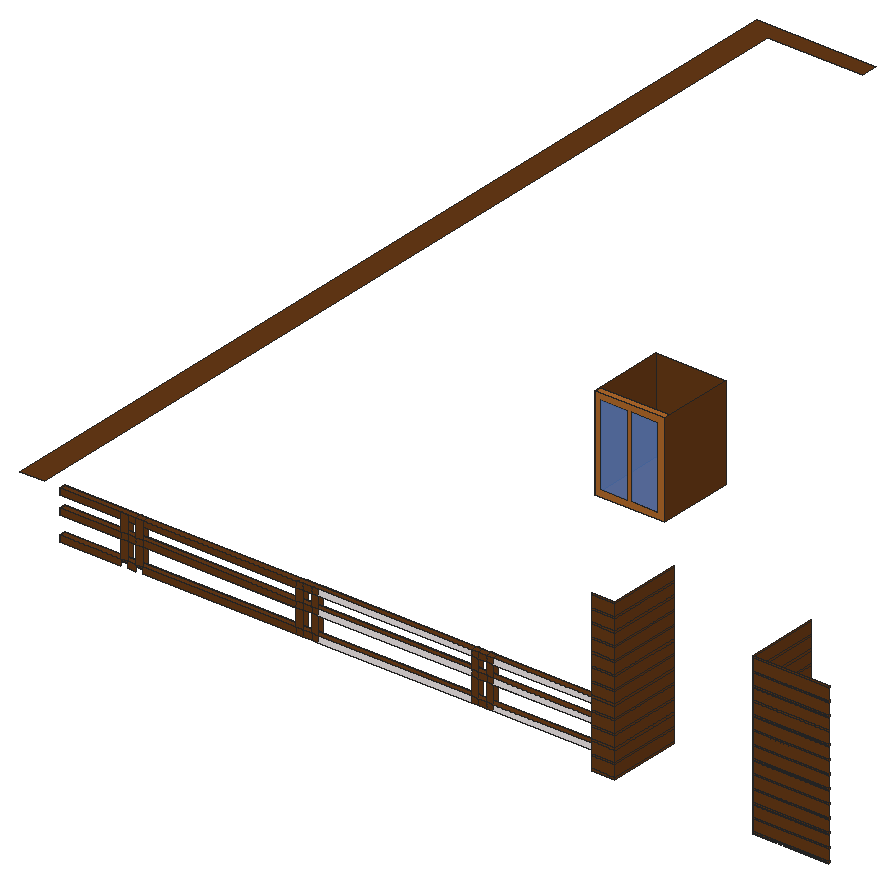
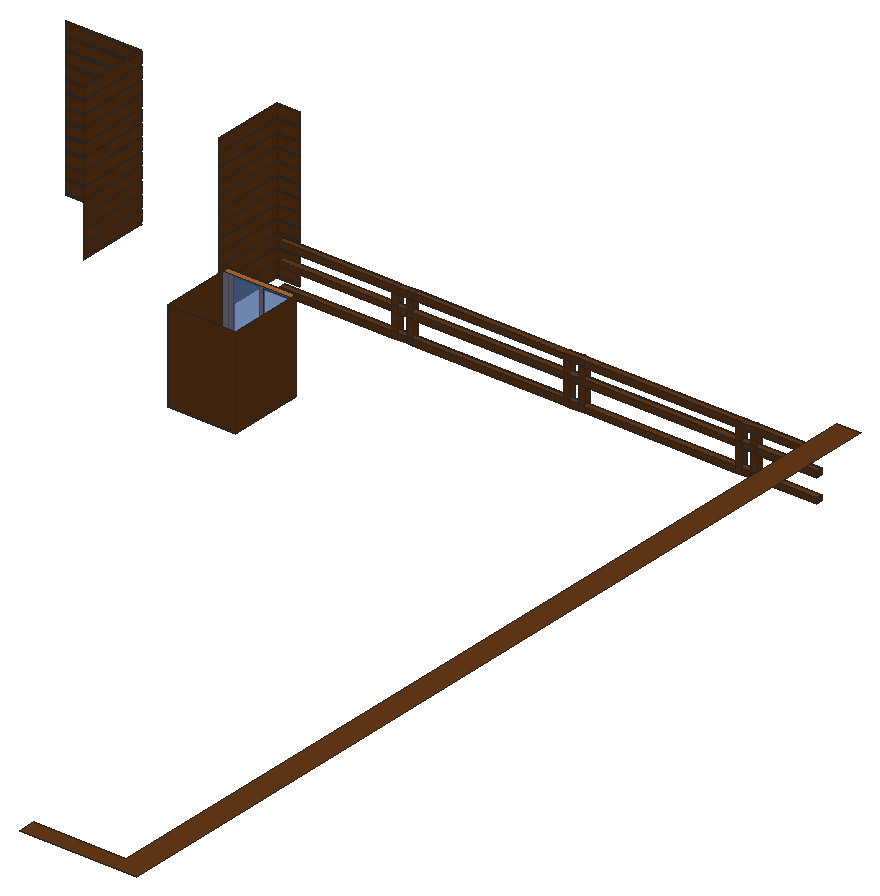
# SketchUp Ruby script. Lengths in inches.
U = 1.inch
M = Sketchup.active_model
def pt(a) = Geom::Point3d.new(a.map { |v| v * U })
def face(e, loops, mat)
  f = e.add_face(loops[0].map { |a| pt(a) })
  loops[1..].each { |l| e.add_face(l.map { |a| pt(a) }).erase! }
  f.material = f.back_material = mat if mat
  f
end
# faces: each face lists its corners as indices into pts; further lists are holes
def faces(e, pts, list, mat = nil) = list.each { |f| face(e, (f[0].is_a?(Array) ? f : [f]).map { |l| l.map { |i| pts[i] } }, mat) }
# xy, xz, yz: faces in a plane at the given z, y or x. An outline is a flat list of corners, or four numbers for a rectangle; further outlines are holes
def ring(l) = l.size == 4 ? [[l[0], l[1]], [l[2], l[1]], [l[2], l[3]], [l[0], l[3]]] : l.each_slice(2).to_a
def flat(e, list, mat, &to3) = list.each { |f| face(e, (f[0].is_a?(Array) ? f : [f]).map { |l| ring(l).map { |u, v| to3.(u, v) } }, mat) }
def xy(e, z, list, mat = nil) = flat(e, list, mat) { |x, y| [x, y, z] }
def xz(e, y, list, mat = nil) = flat(e, list, mat) { |x, z| [x, y, z] }
def yz(e, x, list, mat = nil) = flat(e, list, mat) { |y, z| [x, y, z] }
def lines(e, pts, list) = list.each { |a, b| e.add_line(pt(pts[a]), pt(pts[b])) }
# prism: a flat outline (further loops are holes) pulled along v
def prism(e, loops, v, mat = nil)
  f = face(e, loops, mat); d = Geom::Vector3d.new(v.map { |x| x * U })
  f.pushpull(f.normal.samedirection?(d) ? d.length : -d.length)
end
def box(e, o, s, mat = nil) = prism(e, [[o, [o[0] + s[0], o[1], o[2]], [o[0] + s[0], o[1] + s[1], o[2]], [o[0], o[1] + s[1], o[2]]]], [0, 0, s[2]], mat)
def at(x, y, z, deg = 0) = Geom::Transformation.translation(pt([x, y, z])) * Geom::Transformation.rotation(ORIGIN, Z_AXIS, deg.degrees)
def axes(o, x, y, z) = Geom::Transformation.new([*x, 0, *y, 0, *z, 0, *pt(o).to_a, 1])
def part(name) = M.definitions.add(name)
# library, detail: a bought-in or finely detailed component or shape, given as its bounding box
def library(name, o, s) = part(name).tap { |d| box(d.entities, o, s) }
def detail(e, o, s) = box(e.add_group.entities, o, s)
def put(e, d, t, mat = nil) = e.add_instance(d, t).tap { |i| i.material = mat if mat }
def group(e, t, mat = nil) = e.add_group.tap { |g| g.transformation = t; g.material = mat if mat }.entities
root = M.entities
M.materials.add("Generic").color = [102, 57, 22]
M.materials.add("Generic\#3").color = [243, 235, 235]
M.materials.add("[Translucent Glass Blue]1").color = [100, 149, 237]
M.materials["[Translucent Glass Blue]1"].alpha = 0.5
M.materials.add("[Wood Bamboo]").color = [177, 105, 43]
c1 = part("Group\#5")
xy(c1.entities,0,[[0,0,33.5625,3]],"[Wood Bamboo]")
xy(c1.entities,44.875,[[0,0,33.5625,3]],"[Wood Bamboo]")
xz(c1.entities,0,[[3.04,3.04,15.78,41.84],[17.78,3.04,30.53,41.84]],"[Translucent Glass Blue]1")
xz(c1.entities,0,[[[0,0,33.5625,44.875],[3.04,3.04,15.78,41.84],[17.78,3.04,30.53,41.84]]],"[Wood Bamboo]")
xz(c1.entities,3,[[0,0,33.5625,44.875]],"[Translucent Glass Blue]1")
yz(c1.entities,0,[[0,0,3,44.875]],"[Wood Bamboo]")
yz(c1.entities,33.5625,[[0,0,3,44.875]],"[Wood Bamboo]")
xy(root,296,[[366.12,54.375,377.375,54.68],[377.375,54.375,403,54.68]],"Generic")
xy(root,297,[[366.12,54.375,377.375,54.68],[377.375,54.375,403,54.68]],"Generic")
xy(root,302.3125,[[366.12,54.375,377.375,54.68],[377.375,54.375,403,54.68]],"Generic")
xy(root,303.3125,[[366.12,54.375,377.375,54.68],[377.375,54.375,403,54.68]],"Generic")
xy(root,308.625,[[366.12,54.375,377.375,54.68],[377.375,54.375,403,54.68]],"Generic")
xy(root,309.625,[[366.12,54.375,377.375,54.68],[377.375,54.375,403,54.68]],"Generic")
xy(root,314.9375,[[366.12,54.375,377.375,54.68],[377.375,54.375,403,54.68]],"Generic")
xy(root,315.9375,[[366.12,54.375,377.375,54.68],[377.375,54.375,403,54.68]],"Generic")
xy(root,321.25,[[366.12,54.375,377.375,54.68],[377.375,54.375,403,54.68]],"Generic")
xy(root,321.29,[[54.37,63.57,57.43,66.56],[138.81,63.57,141.87,66.56],[146.12,63.57,149.18,66.56]],"Generic")
xy(root,321.32,[[61.68,63.57,64.75,66.56],[223.25,63.57,226.31,66.56],[230.56,63.57,233.62,66.56]],"Generic")
xy(root,322.25,[[366.12,54.375,377.375,54.68],[377.375,54.375,403,54.68]],"Generic")
xy(root,327.5625,[[366.12,54.375,377.375,54.68],[377.375,54.375,403,54.68]],"Generic")
xy(root,328.375,[[13.1875,54.375,25.02,54.375,25.02,490.0625,70.5625,490.0625,70.5625,498.375,13.1875,498.375]],"Generic")
xy(root,328.5625,[[366.12,54.375,377.375,54.68],[377.375,54.375,403,54.68]],"Generic")
xy(root,331.3125,[[196.46,171.5,230.03,208.375]],"Generic")
xy(root,333.875,[[366.12,54.375,377.375,54.68],[377.375,54.375,403,54.68]],"Generic")
xy(root,334.875,[[366.12,54.375,377.375,54.68],[377.375,54.375,403,54.68]],"Generic")
xy(root,340.1875,[[366.12,54.375,377.375,54.68],[377.375,54.375,403,54.68]],"Generic")
xy(root,341.1875,[[366.12,54.375,377.375,54.68],[377.375,54.375,403,54.68]],"Generic")
xy(root,346.5,[[366.12,54.375,377.375,54.68],[377.375,54.375,403,54.68]],"Generic")
xy(root,347.5,[[366.12,54.375,377.375,54.68],[377.375,54.375,403,54.68]],"Generic")
xy(root,359.125,[[366.12,54.375,377.375,54.68],[377.375,54.375,403,54.68]],"Generic")
xy(root,360.125,[[366.12,54.375,377.375,54.68],[377.375,54.375,403,54.68]],"Generic")
xy(root,365.4375,[[366.12,54.375,377.375,54.68],[377.375,54.375,403,54.68]],"Generic")
xy(root,366.4375,[[366.12,54.375,377.375,54.68],[377.375,54.375,403,54.68]],"Generic")
xy(root,371.75,[[366.12,54.375,377.375,54.68],[377.375,54.375,403,54.68]],"Generic")
xz(root,54.375,[[288.56,296,299.81,297],[288.56,297,299.81,302.3125],[366.12,297,403,302.3125],[288.56,302.3125,299.81,303.3125],[288.56,303.3125,299.81,308.625],
  [366.12,303.3125,403,308.625],[288.56,308.625,299.81,309.625],[288.56,309.625,299.81,314.9375],[366.12,309.625,403,314.9375],[288.56,314.9375,299.81,315.9375],
  [288.56,315.9375,299.81,321.25],[366.12,315.9375,403,321.25],[288.56,321.25,299.81,322.25],[288.56,322.25,299.81,327.5625],[366.12,322.25,403,327.5625],
  [288.56,327.5625,299.81,328.5625],[288.56,328.5625,299.81,333.875],[366.12,328.5625,403,333.875],[288.56,333.875,299.81,334.875],[288.56,334.875,299.81,340.1875],
  [366.12,334.875,403,340.1875],[288.56,340.1875,299.81,341.1875],[288.56,341.1875,299.81,346.5],[366.12,341.1875,403,346.5],[288.56,346.5,299.81,347.5],
  [288.56,347.5,299.81,352.8125],[366.12,347.5,403,352.8125],[288.56,352.8125,299.81,353.8125],[366.12,352.8125,403,353.8125],[288.56,353.8125,299.81,359.125],
  [366.12,353.8125,403,359.125],[288.56,359.125,299.81,360.125],[288.56,360.125,299.81,365.4375],[366.12,360.125,403,365.4375],[288.56,365.4375,299.81,366.4375],
  [288.56,366.4375,299.81,371.75],[366.12,366.4375,403,371.75],[288.56,371.75,299.81,372.75]],"Generic")
xz(root,54.68,[[366.12,296,403,297],[366.12,302.3125,403,303.3125],[366.12,308.625,403,309.625],[366.12,314.9375,403,315.9375],[366.12,321.25,403,322.25],
  [366.12,327.5625,403,328.5625],[366.12,333.875,403,334.875],[366.12,340.1875,403,341.1875],[366.12,346.5,403,347.5],[366.12,359.125,403,360.125],
  [366.12,365.4375,403,366.4375],[366.12,371.75,403,372.75]],"Generic")
xz(root,63.57,[[25.02,298.26,54.37,301.19],[57.43,298.26,61.68,301.19],[64.75,298.26,138.81,301.19],[138.81,298.26,141.87,301.19],[141.87,298.26,146.12,301.19],
  [146.12,298.26,149.18,301.19],[223.25,298.26,226.31,301.19],[226.31,298.26,230.56,301.19],[230.56,298.26,233.62,301.19],[54.37,301.19,57.43,309.82],
  [61.68,301.19,64.75,309.82],[138.81,301.19,141.87,309.82],[146.12,301.19,149.18,309.82],[223.25,301.19,226.31,309.82],[230.56,301.19,233.62,309.82],
  [25.02,309.82,54.37,312.76],[54.37,309.82,57.43,312.76],[57.43,309.82,61.68,312.76],[61.68,309.82,64.75,312.76],[64.75,309.82,138.81,312.76],
  [138.81,309.82,141.87,312.76],[141.87,309.82,146.12,312.76],[146.12,309.82,149.18,312.76],[223.25,309.82,226.31,312.76],[226.31,309.82,230.56,312.76],
  [230.56,309.82,233.62,312.76],[54.37,312.76,57.43,321.29],[61.68,312.76,64.75,321.32],[138.81,312.76,141.87,318.38],[146.12,312.76,149.18,318.38],
  [223.25,312.76,226.31,318.38],[230.56,312.76,233.62,318.38],[25.02,318.38,54.37,321.32],[57.43,318.38,61.68,321.32],[64.75,318.38,138.81,321.32],
  [138.81,318.38,141.87,321.29],[141.87,318.38,146.12,321.32],[146.12,318.38,149.18,321.29],[223.25,318.38,226.31,321.32],[226.31,318.38,230.56,321.32],
  [230.56,318.38,233.62,321.32],[54.37,321.29,57.43,321.32],[138.81,321.29,141.87,321.32],[146.12,321.29,149.18,321.32]],"Generic")
xz(root,63.57,[[149.18,298.26,223.25,301.19],[233.62,298.26,288.56,301.19],[149.18,309.82,223.25,312.76],[233.62,309.82,288.56,312.76],[149.18,318.38,223.25,321.32],
  [233.62,318.38,288.56,321.32]],"Generic\#3")
xz(root,66.56,[[25.02,298.23,54.37,301.17],[54.37,298.23,57.43,301.17],[57.43,298.23,61.68,301.17],[61.68,298.23,64.75,301.17],[64.75,298.23,138.81,301.17],
  [138.81,298.23,141.87,301.17],[141.87,298.23,146.12,301.17],[146.12,298.23,149.18,301.17],[149.18,298.23,223.25,301.17],[223.25,298.23,226.31,301.17],
  [226.31,298.23,230.56,301.17],[230.56,298.23,233.62,301.17],[233.62,298.23,288.56,301.17],[54.37,301.17,57.43,309.79],[61.68,301.17,64.75,309.79],
  [138.81,301.17,141.87,309.79],[146.12,301.17,149.18,309.79],[223.25,301.17,226.31,309.79],[230.56,301.17,233.62,309.79],[25.02,309.79,54.37,312.73],
  [54.37,309.79,57.43,312.73],[57.43,309.79,61.68,312.73],[61.68,309.79,64.75,312.73],[64.75,309.79,138.81,312.73],[138.81,309.79,141.87,312.73],
  [141.87,309.79,146.12,312.73],[146.12,309.79,149.18,312.73],[149.18,309.79,223.25,312.73],[223.25,309.79,226.31,312.73],[226.31,309.79,230.56,312.73],
  [230.56,309.79,233.62,312.73],[233.62,309.79,288.56,312.73],[54.37,312.73,57.43,318.36],[61.68,312.73,64.75,318.36],[138.81,312.73,141.87,318.36],
  [146.12,312.73,149.18,318.36],[223.25,312.73,226.31,318.36],[230.56,312.73,233.62,318.36],[25.02,318.36,54.37,321.29],[54.37,318.36,57.43,321.29],
  [57.43,318.36,61.68,321.29],[61.68,318.36,64.75,321.29],[64.75,318.36,138.81,321.29],[138.81,318.36,141.87,321.29],[141.87,318.36,146.12,321.29],
  [146.12,318.36,149.18,321.29],[149.18,318.36,223.25,321.29],[223.25,318.36,226.31,321.29],[226.31,318.36,230.56,321.29],[230.56,318.36,233.62,321.29],
  [233.62,318.36,288.56,321.29],[61.68,321.29,64.75,321.32],[223.25,321.29,226.31,321.32],[230.56,321.29,233.62,321.32]],"Generic")
xz(root,208.375,[[196.46,331.3125,230.03,376.1875]],"Generic")
yz(root,25.02,[[66.56,298.23,63.57,298.26,63.57,301.19,66.56,301.17],[66.56,309.79,63.57,309.82,63.57,312.76,66.56,312.73],[66.56,318.36,63.57,318.38,63.57,321.32,66.56,321.29]],"Generic")
yz(root,196.46,[[171.5,331.3125,208.375,376.1875]],"Generic")
yz(root,230.03,[[171.5,331.3125,208.375,376.1875]],"Generic")
yz(root,299.81,[[54.375,296,89.74,297],[54.375,297,89.74,302.3125],[54.375,302.3125,89.74,303.3125],[54.375,303.3125,89.74,308.625],[54.375,308.625,89.74,309.625],
  [54.375,309.625,89.74,314.9375],[54.375,314.9375,89.74,315.9375],[54.375,315.9375,89.74,321.25],[54.375,321.25,89.74,322.25],[54.375,322.25,89.74,327.5625],
  [54.375,327.5625,89.74,328.5625],[54.375,328.5625,89.74,333.875],[54.375,333.875,89.74,334.875],[54.375,334.875,89.74,340.1875],[54.375,340.1875,89.74,341.1875],
  [54.375,341.1875,89.74,346.5],[54.375,346.5,89.74,347.5],[54.375,347.5,89.74,352.8125],[54.375,352.8125,89.74,353.8125],[54.375,353.8125,89.74,359.125],
  [54.375,359.125,89.74,360.125],[54.375,360.125,89.74,365.4375],[54.375,365.4375,89.74,366.4375],[54.375,366.4375,89.74,371.75],[54.375,371.75,89.74,372.75]],"Generic")
yz(root,366.12,[[54.68,296,89.74,297],[54.375,297,89.74,302.3125],[54.68,302.3125,89.74,303.3125],[54.375,303.3125,89.74,308.625],[54.68,308.625,89.74,309.625],
  [54.375,309.625,89.74,314.9375],[54.68,314.9375,89.74,315.9375],[54.375,315.9375,89.74,321.25],[54.68,321.25,89.74,322.25],[54.375,322.25,89.74,327.5625],
  [54.68,327.5625,89.74,328.5625],[54.375,328.5625,89.74,333.875],[54.68,333.875,89.74,334.875],[54.375,334.875,89.74,340.1875],[54.68,340.1875,89.74,341.1875],
  [54.375,341.1875,89.74,346.5],[54.68,346.5,89.74,347.5],[54.375,347.5,89.74,352.8125],[54.375,352.8125,89.74,353.8125],[54.375,353.8125,89.74,359.125],
  [54.68,359.125,89.74,360.125],[54.375,360.125,89.74,365.4375],[54.68,365.4375,89.74,366.4375],[54.375,366.4375,89.74,371.75],[54.68,371.75,89.74,372.75]],"Generic")
yz(root,403,[[54.375,296,54.68,297],[54.375,302.3125,54.68,303.3125],[54.375,308.625,54.68,309.625],[54.375,314.9375,54.68,315.9375],[54.375,321.25,54.68,322.25],
  [54.375,327.5625,54.68,328.5625],[54.375,333.875,54.68,334.875],[54.375,340.1875,54.68,341.1875],[54.375,346.5,54.68,347.5],[54.375,359.125,54.68,360.125],
  [54.375,365.4375,54.68,366.4375],[54.375,371.75,54.68,372.75]],"Generic")
p = [[25.02,66.56,301.17],[25.02,63.57,301.19],[54.37,63.57,301.19],[57.43,63.57,301.19],[61.68,63.57,301.19],[64.75,63.57,301.19],
  [138.81,63.57,301.19],[141.87,63.57,301.19],[146.12,63.57,301.19],[149.18,63.57,301.19],[223.25,63.57,301.19],[226.31,63.57,301.19],
  [230.56,63.57,301.19],[233.62,63.57,301.19],[288.56,63.57,301.19],[288.56,66.56,301.17],[233.62,66.56,301.17],[230.56,66.56,301.17],
  [226.31,66.56,301.17],[223.25,66.56,301.17],[149.18,66.56,301.17],[146.12,66.56,301.17],[141.87,66.56,301.17],[138.81,66.56,301.17],
  [64.75,66.56,301.17],[61.68,66.56,301.17],[57.43,66.56,301.17],[54.37,66.56,301.17],[25.02,63.57,309.82],[25.02,66.56,309.79],
  [54.37,66.56,309.79],[57.43,66.56,309.79],[61.68,66.56,309.79],[64.75,66.56,309.79],[138.81,66.56,309.79],[141.87,66.56,309.79],
  [146.12,66.56,309.79],[149.18,66.56,309.79],[223.25,66.56,309.79],[226.31,66.56,309.79],[230.56,66.56,309.79],[233.62,66.56,309.79],
  [288.56,66.56,309.79],[288.56,63.57,309.82],[233.62,63.57,309.82],[230.56,63.57,309.82],[226.31,63.57,309.82],[223.25,63.57,309.82],
  [149.18,63.57,309.82],[146.12,63.57,309.82],[141.87,63.57,309.82],[138.81,63.57,309.82],[64.75,63.57,309.82],[61.68,63.57,309.82],
  [57.43,63.57,309.82],[54.37,63.57,309.82],[25.02,66.56,312.73],[25.02,63.57,312.76],[54.37,63.57,312.76],[57.43,63.57,312.76],
  [61.68,63.57,312.76],[64.75,63.57,312.76],[138.81,63.57,312.76],[141.87,63.57,312.76],[146.12,63.57,312.76],[149.18,63.57,312.76],
  [223.25,63.57,312.76],[226.31,63.57,312.76],[230.56,63.57,312.76],[233.62,63.57,312.76],[288.56,63.57,312.76],[288.56,66.56,312.73],
  [233.62,66.56,312.73],[230.56,66.56,312.73],[226.31,66.56,312.73],[223.25,66.56,312.73],[149.18,66.56,312.73],[146.12,66.56,312.73],
  [141.87,66.56,312.73],[138.81,66.56,312.73],[64.75,66.56,312.73],[61.68,66.56,312.73],[57.43,66.56,312.73],[54.37,66.56,312.73],
  [25.02,66.56,321.29],[25.02,63.57,321.32],[54.37,63.57,321.32],[57.43,63.57,321.32],[61.68,63.57,321.32],[64.75,63.57,321.32],
  [138.81,63.57,321.32],[141.87,63.57,321.32],[146.12,63.57,321.32],[149.18,63.57,321.32],[223.25,63.57,321.32],[226.31,63.57,321.32],
  [230.56,63.57,321.32],[233.62,63.57,321.32],[288.56,63.57,321.32],[288.56,66.56,321.29],[233.62,66.56,321.29],[230.56,66.56,321.29],
  [226.31,66.56,321.29],[223.25,66.56,321.29],[149.18,66.56,321.29],[146.12,66.56,321.29],[141.87,66.56,321.29],[138.81,66.56,321.29],
  [64.75,66.56,321.29],[61.68,66.56,321.29],[57.43,66.56,321.29],[54.37,66.56,321.29],[25.02,65.08,319.82],[288.56,65.08,319.82],
  [25.02,65.08,311.07],[288.56,65.08,311.07],[25.02,65.08,299.32],[288.56,65.08,299.32]]
faces(root,p,[[0,1,2,3,4,5,6,7,8,9,10,11,12,13,14,15,16,17,18,19,20,21,22,23,24,25,26,27],[28,29,30,31,32,33,34,35,36,37,38,39,40,41,42,43,44,45,46,47,48,49,50,51,52,53,54,55],[56,57,58,59,60,61,62,63,64,65,66,67,68,69,70,71,72,73,74,75,76,77,78,79,80,81,82,83],[84,85,86,87,88,89,90,91,92,93,94,95,96,97,98,99,100,101,102,103,104,105,106,107,108,109,110,111]],"Generic")
lines(root,p,[[112,113],[114,115],[116,117]])
put(root,c1,at(196.46,171.5,331.3125))
